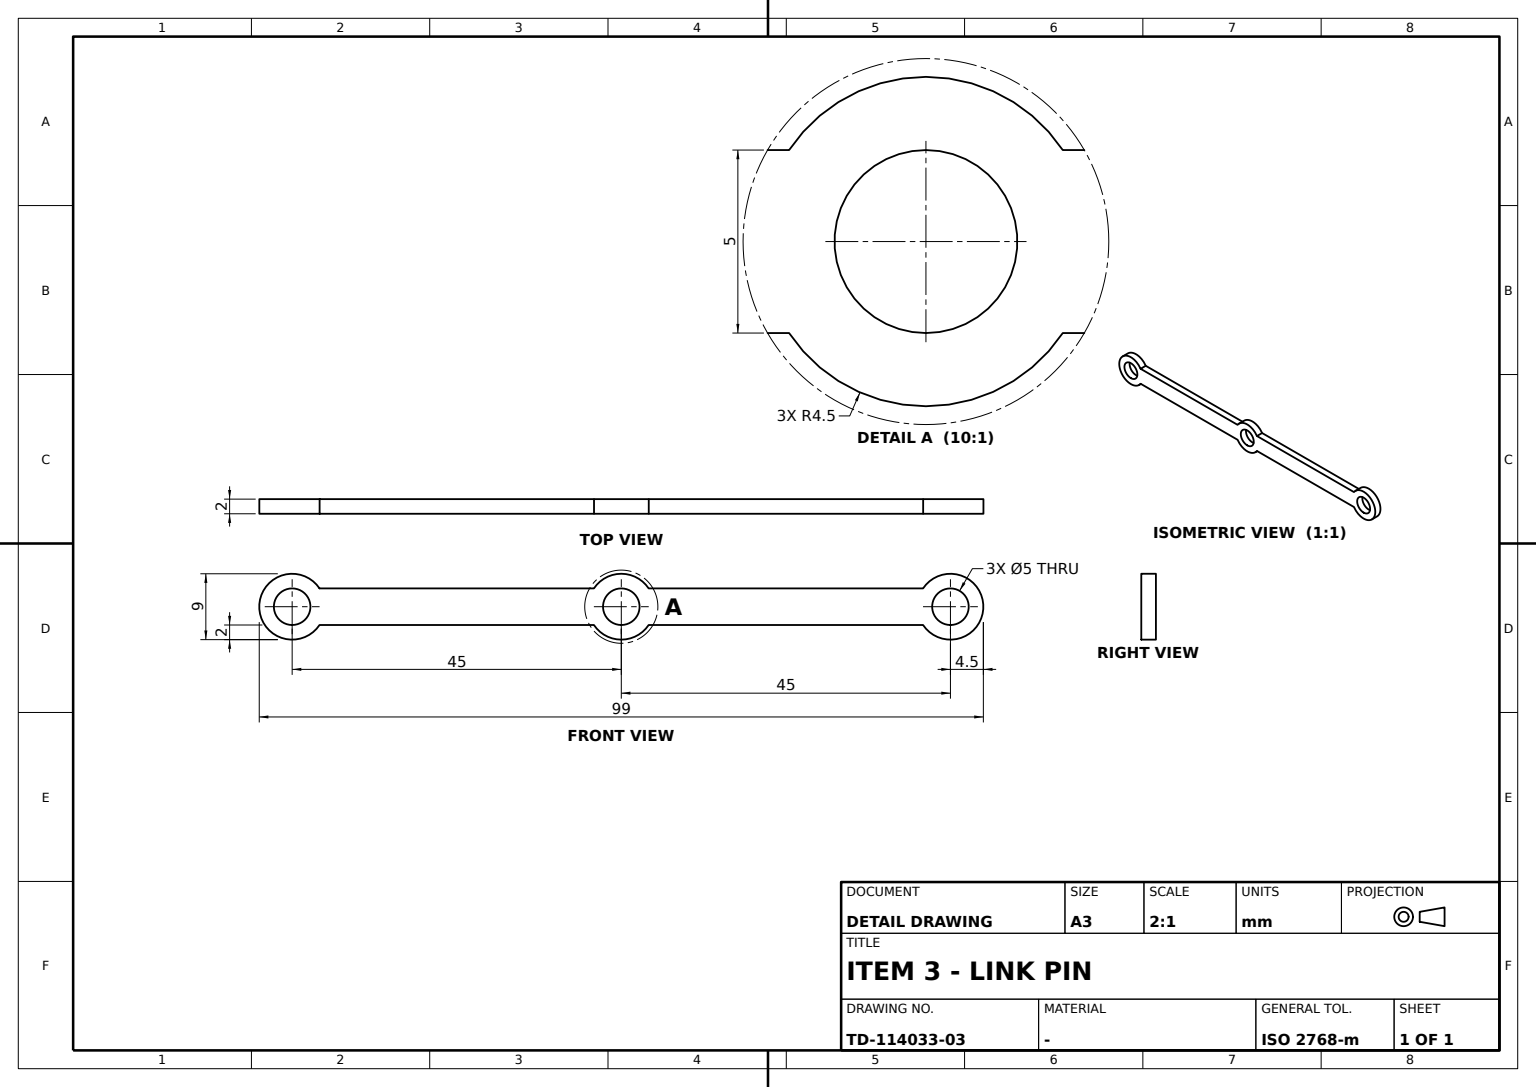
ISO-10303-21;
HEADER;
FILE_DESCRIPTION((''),'2;1');
FILE_NAME('','',(''),(''),'','','');
FILE_SCHEMA(('AUTOMOTIVE_DESIGN'));
ENDSEC;
DATA;
#1=APPLICATION_CONTEXT('');
#2=PRODUCT_CONTEXT('',#1,'mechanical');
#3=PRODUCT('','','',(#2));
#4=PRODUCT_DEFINITION_FORMATION('','',#3);
#5=PRODUCT_DEFINITION_CONTEXT('',#1,'design');
#6=PRODUCT_DEFINITION('','',#4,#5);
#7=PRODUCT_DEFINITION_SHAPE('','',#6);
#8=(LENGTH_UNIT()NAMED_UNIT(*)SI_UNIT(.MILLI.,.METRE.));
#9=(NAMED_UNIT(*)PLANE_ANGLE_UNIT()SI_UNIT($,.RADIAN.));
#10=(NAMED_UNIT(*)SI_UNIT($,.STERADIAN.)SOLID_ANGLE_UNIT());
#11=UNCERTAINTY_MEASURE_WITH_UNIT(LENGTH_MEASURE(0.005),#8,'distance_accuracy_value','');
#12=(GEOMETRIC_REPRESENTATION_CONTEXT(3)GLOBAL_UNCERTAINTY_ASSIGNED_CONTEXT((#11))GLOBAL_UNIT_ASSIGNED_CONTEXT((#8,#9,#10))REPRESENTATION_CONTEXT('',''));
#13=CARTESIAN_POINT('',(-1.,3.741657,-2.5));
#14=VERTEX_POINT('',#13);
#15=CARTESIAN_POINT('',(-1.,41.258343,-2.5));
#16=VERTEX_POINT('',#15);
#17=CARTESIAN_POINT('',(-1.,0.,-2.5));
#18=DIRECTION('',(0.,1.,0.));
#19=VECTOR('',#18,1000.);
#20=LINE('',#17,#19);
#21=EDGE_CURVE('',#14,#16,#20,.T.);
#22=ORIENTED_EDGE('',*,*,#21,.T.);
#23=CARTESIAN_POINT('',(1.,41.258343,-2.5));
#24=VERTEX_POINT('',#23);
#25=DIRECTION('',(1.,0.,0.));
#26=VECTOR('',#25,1000.);
#27=LINE('',#15,#26);
#28=EDGE_CURVE('',#16,#24,#27,.T.);
#29=ORIENTED_EDGE('',*,*,#28,.T.);
#30=CARTESIAN_POINT('',(1.,3.741657,-2.5));
#31=VERTEX_POINT('',#30);
#32=CARTESIAN_POINT('',(1.,0.,-2.5));
#33=LINE('',#32,#19);
#34=EDGE_CURVE('',#31,#24,#33,.T.);
#35=ORIENTED_EDGE('',*,*,#34,.F.);
#36=LINE('',#13,#26);
#37=EDGE_CURVE('',#14,#31,#36,.T.);
#38=ORIENTED_EDGE('',*,*,#37,.F.);
#39=EDGE_LOOP('',(#22,#29,#35,#38));
#40=FACE_BOUND('',#39,.T.);
#41=CARTESIAN_POINT('',(0.,-41.258343,-2.5));
#42=DIRECTION('',(0.,0.,-1.));
#43=AXIS2_PLACEMENT_3D('',#41,#42,#18);
#44=PLANE('',#43);
#45=ADVANCED_FACE('',(#40),#44,.T.);
#46=CARTESIAN_POINT('',(-1.,-41.258343,2.5));
#47=VERTEX_POINT('',#46);
#48=CARTESIAN_POINT('',(-1.,-41.258343,-2.5));
#49=VERTEX_POINT('',#48);
#50=CARTESIAN_POINT('',(-1.,-45.,0.));
#51=AXIS2_PLACEMENT_3D('',#50,#25,#42);
#52=CIRCLE('',#51,4.5);
#53=EDGE_CURVE('',#47,#49,#52,.T.);
#54=ORIENTED_EDGE('',*,*,#53,.T.);
#55=CARTESIAN_POINT('',(1.,-41.258343,-2.5));
#56=VERTEX_POINT('',#55);
#57=LINE('',#48,#26);
#58=EDGE_CURVE('',#49,#56,#57,.T.);
#59=ORIENTED_EDGE('',*,*,#58,.T.);
#60=CARTESIAN_POINT('',(1.,-41.258343,2.5));
#61=VERTEX_POINT('',#60);
#62=CARTESIAN_POINT('',(1.,-45.,0.));
#63=AXIS2_PLACEMENT_3D('',#62,#25,#42);
#64=CIRCLE('',#63,4.5);
#65=EDGE_CURVE('',#61,#56,#64,.T.);
#66=ORIENTED_EDGE('',*,*,#65,.F.);
#67=LINE('',#46,#26);
#68=EDGE_CURVE('',#47,#61,#67,.T.);
#69=ORIENTED_EDGE('',*,*,#68,.F.);
#70=EDGE_LOOP('',(#54,#59,#66,#69));
#71=FACE_BOUND('',#70,.T.);
#72=CARTESIAN_POINT('',(0.,-45.,0.));
#73=AXIS2_PLACEMENT_3D('',#72,#25,#18);
#74=CYLINDRICAL_SURFACE('',#73,4.5);
#75=ADVANCED_FACE('',(#71),#74,.T.);
#76=CARTESIAN_POINT('',(-1.,-3.741657,-2.5));
#77=VERTEX_POINT('',#76);
#78=CARTESIAN_POINT('',(1.,-3.741657,-2.5));
#79=VERTEX_POINT('',#78);
#80=LINE('',#76,#26);
#81=EDGE_CURVE('',#77,#79,#80,.T.);
#82=ORIENTED_EDGE('',*,*,#81,.F.);
#83=CARTESIAN_POINT('',(-1.,0.,0.));
#84=AXIS2_PLACEMENT_3D('',#83,#25,#42);
#85=CIRCLE('',#84,4.5);
#86=EDGE_CURVE('',#77,#14,#85,.T.);
#87=ORIENTED_EDGE('',*,*,#86,.T.);
#88=ORIENTED_EDGE('',*,*,#37,.T.);
#89=CARTESIAN_POINT('',(1.,0.,0.));
#90=AXIS2_PLACEMENT_3D('',#89,#25,#42);
#91=CIRCLE('',#90,4.5);
#92=EDGE_CURVE('',#79,#31,#91,.T.);
#93=ORIENTED_EDGE('',*,*,#92,.F.);
#94=EDGE_LOOP('',(#82,#87,#88,#93));
#95=FACE_BOUND('',#94,.T.);
#96=CARTESIAN_POINT('',(0.,0.,0.));
#97=AXIS2_PLACEMENT_3D('',#96,#25,#18);
#98=CYLINDRICAL_SURFACE('',#97,4.5);
#99=ADVANCED_FACE('',(#95),#98,.T.);
#100=CARTESIAN_POINT('',(-1.,-3.741657,2.5));
#101=VERTEX_POINT('',#100);
#102=CARTESIAN_POINT('',(1.,-3.741657,2.5));
#103=VERTEX_POINT('',#102);
#104=LINE('',#100,#26);
#105=EDGE_CURVE('',#101,#103,#104,.T.);
#106=ORIENTED_EDGE('',*,*,#105,.T.);
#107=CARTESIAN_POINT('',(1.,3.741657,2.5));
#108=VERTEX_POINT('',#107);
#109=EDGE_CURVE('',#108,#103,#91,.T.);
#110=ORIENTED_EDGE('',*,*,#109,.F.);
#111=CARTESIAN_POINT('',(-1.,3.741657,2.5));
#112=VERTEX_POINT('',#111);
#113=LINE('',#111,#26);
#114=EDGE_CURVE('',#112,#108,#113,.T.);
#115=ORIENTED_EDGE('',*,*,#114,.F.);
#116=EDGE_CURVE('',#112,#101,#85,.T.);
#117=ORIENTED_EDGE('',*,*,#116,.T.);
#118=EDGE_LOOP('',(#106,#110,#115,#117));
#119=FACE_BOUND('',#118,.T.);
#120=ADVANCED_FACE('',(#119),#98,.T.);
#121=VERTEX_POINT('',#17);
#122=CIRCLE('',#84,2.5);
#123=EDGE_CURVE('',#121,#121,#122,.T.);
#124=ORIENTED_EDGE('',*,*,#123,.F.);
#125=EDGE_LOOP('',(#124));
#126=FACE_BOUND('',#125,.T.);
#127=VERTEX_POINT('',#32);
#128=CIRCLE('',#90,2.5);
#129=EDGE_CURVE('',#127,#127,#128,.T.);
#130=ORIENTED_EDGE('',*,*,#129,.T.);
#131=EDGE_LOOP('',(#130));
#132=FACE_BOUND('',#131,.T.);
#133=CYLINDRICAL_SURFACE('',#97,2.5);
#134=ADVANCED_FACE('',(#126,#132),#133,.F.);
#135=CARTESIAN_POINT('',(1.,45.,-2.5));
#136=VERTEX_POINT('',#135);
#137=CARTESIAN_POINT('',(1.,45.,0.));
#138=AXIS2_PLACEMENT_3D('',#137,#25,#42);
#139=CIRCLE('',#138,2.5);
#140=EDGE_CURVE('',#136,#136,#139,.T.);
#141=ORIENTED_EDGE('',*,*,#140,.F.);
#142=EDGE_LOOP('',(#141));
#143=FACE_BOUND('',#142,.T.);
#144=ORIENTED_EDGE('',*,*,#92,.T.);
#145=ORIENTED_EDGE('',*,*,#34,.T.);
#146=CARTESIAN_POINT('',(1.,41.258343,2.5));
#147=VERTEX_POINT('',#146);
#148=CIRCLE('',#138,4.5);
#149=EDGE_CURVE('',#24,#147,#148,.T.);
#150=ORIENTED_EDGE('',*,*,#149,.T.);
#151=CARTESIAN_POINT('',(1.,0.,2.5));
#152=LINE('',#151,#19);
#153=EDGE_CURVE('',#108,#147,#152,.T.);
#154=ORIENTED_EDGE('',*,*,#153,.F.);
#155=ORIENTED_EDGE('',*,*,#109,.T.);
#156=EDGE_CURVE('',#61,#103,#152,.T.);
#157=ORIENTED_EDGE('',*,*,#156,.F.);
#158=ORIENTED_EDGE('',*,*,#65,.T.);
#159=EDGE_CURVE('',#56,#79,#33,.T.);
#160=ORIENTED_EDGE('',*,*,#159,.T.);
#161=EDGE_LOOP('',(#144,#145,#150,#154,#155,#157,#158,#160));
#162=FACE_BOUND('',#161,.T.);
#163=CARTESIAN_POINT('',(1.,-45.,-2.5));
#164=VERTEX_POINT('',#163);
#165=CIRCLE('',#63,2.5);
#166=EDGE_CURVE('',#164,#164,#165,.T.);
#167=ORIENTED_EDGE('',*,*,#166,.F.);
#168=EDGE_LOOP('',(#167));
#169=FACE_BOUND('',#168,.T.);
#170=ORIENTED_EDGE('',*,*,#129,.F.);
#171=EDGE_LOOP('',(#170));
#172=FACE_BOUND('',#171,.T.);
#173=AXIS2_PLACEMENT_3D('',#89,#25,#18);
#174=PLANE('',#173);
#175=ADVANCED_FACE('',(#143,#162,#169,#172),#174,.T.);
#176=ORIENTED_EDGE('',*,*,#68,.T.);
#177=ORIENTED_EDGE('',*,*,#156,.T.);
#178=ORIENTED_EDGE('',*,*,#105,.F.);
#179=CARTESIAN_POINT('',(-1.,0.,2.5));
#180=LINE('',#179,#19);
#181=EDGE_CURVE('',#47,#101,#180,.T.);
#182=ORIENTED_EDGE('',*,*,#181,.F.);
#183=EDGE_LOOP('',(#176,#177,#178,#182));
#184=FACE_BOUND('',#183,.T.);
#185=CARTESIAN_POINT('',(0.,3.741657,2.5));
#186=AXIS2_PLACEMENT_3D('',#185,#42,#18);
#187=PLANE('',#186);
#188=ADVANCED_FACE('',(#184),#187,.F.);
#189=CARTESIAN_POINT('',(-1.,41.258343,2.5));
#190=VERTEX_POINT('',#189);
#191=LINE('',#189,#26);
#192=EDGE_CURVE('',#190,#147,#191,.T.);
#193=ORIENTED_EDGE('',*,*,#192,.T.);
#194=ORIENTED_EDGE('',*,*,#149,.F.);
#195=ORIENTED_EDGE('',*,*,#28,.F.);
#196=CARTESIAN_POINT('',(-1.,45.,0.));
#197=AXIS2_PLACEMENT_3D('',#196,#25,#42);
#198=CIRCLE('',#197,4.5);
#199=EDGE_CURVE('',#16,#190,#198,.T.);
#200=ORIENTED_EDGE('',*,*,#199,.T.);
#201=EDGE_LOOP('',(#193,#194,#195,#200));
#202=FACE_BOUND('',#201,.T.);
#203=CARTESIAN_POINT('',(0.,45.,0.));
#204=AXIS2_PLACEMENT_3D('',#203,#25,#18);
#205=CYLINDRICAL_SURFACE('',#204,4.5);
#206=ADVANCED_FACE('',(#202),#205,.T.);
#207=EDGE_CURVE('',#112,#190,#180,.T.);
#208=ORIENTED_EDGE('',*,*,#207,.F.);
#209=ORIENTED_EDGE('',*,*,#114,.T.);
#210=ORIENTED_EDGE('',*,*,#153,.T.);
#211=ORIENTED_EDGE('',*,*,#192,.F.);
#212=EDGE_LOOP('',(#208,#209,#210,#211));
#213=FACE_BOUND('',#212,.T.);
#214=ADVANCED_FACE('',(#213),#187,.F.);
#215=ORIENTED_EDGE('',*,*,#58,.F.);
#216=EDGE_CURVE('',#49,#77,#20,.T.);
#217=ORIENTED_EDGE('',*,*,#216,.T.);
#218=ORIENTED_EDGE('',*,*,#81,.T.);
#219=ORIENTED_EDGE('',*,*,#159,.F.);
#220=EDGE_LOOP('',(#215,#217,#218,#219));
#221=FACE_BOUND('',#220,.T.);
#222=ADVANCED_FACE('',(#221),#44,.T.);
#223=CARTESIAN_POINT('',(-1.,-45.,-2.5));
#224=VERTEX_POINT('',#223);
#225=CIRCLE('',#51,2.5);
#226=EDGE_CURVE('',#224,#224,#225,.T.);
#227=ORIENTED_EDGE('',*,*,#226,.F.);
#228=EDGE_LOOP('',(#227));
#229=FACE_BOUND('',#228,.T.);
#230=ORIENTED_EDGE('',*,*,#166,.T.);
#231=EDGE_LOOP('',(#230));
#232=FACE_BOUND('',#231,.T.);
#233=CYLINDRICAL_SURFACE('',#73,2.5);
#234=ADVANCED_FACE('',(#229,#232),#233,.F.);
#235=ORIENTED_EDGE('',*,*,#140,.T.);
#236=EDGE_LOOP('',(#235));
#237=FACE_BOUND('',#236,.T.);
#238=CARTESIAN_POINT('',(-1.,45.,-2.5));
#239=VERTEX_POINT('',#238);
#240=CIRCLE('',#197,2.5);
#241=EDGE_CURVE('',#239,#239,#240,.T.);
#242=ORIENTED_EDGE('',*,*,#241,.F.);
#243=EDGE_LOOP('',(#242));
#244=FACE_BOUND('',#243,.T.);
#245=CYLINDRICAL_SURFACE('',#204,2.5);
#246=ADVANCED_FACE('',(#237,#244),#245,.F.);
#247=ORIENTED_EDGE('',*,*,#241,.T.);
#248=EDGE_LOOP('',(#247));
#249=FACE_BOUND('',#248,.T.);
#250=ORIENTED_EDGE('',*,*,#86,.F.);
#251=ORIENTED_EDGE('',*,*,#216,.F.);
#252=ORIENTED_EDGE('',*,*,#53,.F.);
#253=ORIENTED_EDGE('',*,*,#181,.T.);
#254=ORIENTED_EDGE('',*,*,#116,.F.);
#255=ORIENTED_EDGE('',*,*,#207,.T.);
#256=ORIENTED_EDGE('',*,*,#199,.F.);
#257=ORIENTED_EDGE('',*,*,#21,.F.);
#258=EDGE_LOOP('',(#250,#251,#252,#253,#254,#255,#256,#257));
#259=FACE_BOUND('',#258,.T.);
#260=ORIENTED_EDGE('',*,*,#123,.T.);
#261=EDGE_LOOP('',(#260));
#262=FACE_BOUND('',#261,.T.);
#263=ORIENTED_EDGE('',*,*,#226,.T.);
#264=EDGE_LOOP('',(#263));
#265=FACE_BOUND('',#264,.T.);
#266=AXIS2_PLACEMENT_3D('',#83,#25,#18);
#267=PLANE('',#266);
#268=ADVANCED_FACE('',(#249,#259,#262,#265),#267,.F.);
#269=CLOSED_SHELL('',(#45,#75,#99,#120,#134,#175,#188,#206,#214,#222,#234,#246,#268));
#270=MANIFOLD_SOLID_BREP('',#269);
#271=ADVANCED_BREP_SHAPE_REPRESENTATION('',(#270),#12);
#272=SHAPE_DEFINITION_REPRESENTATION(#7,#271);
ENDSEC;
END-ISO-10303-21;
